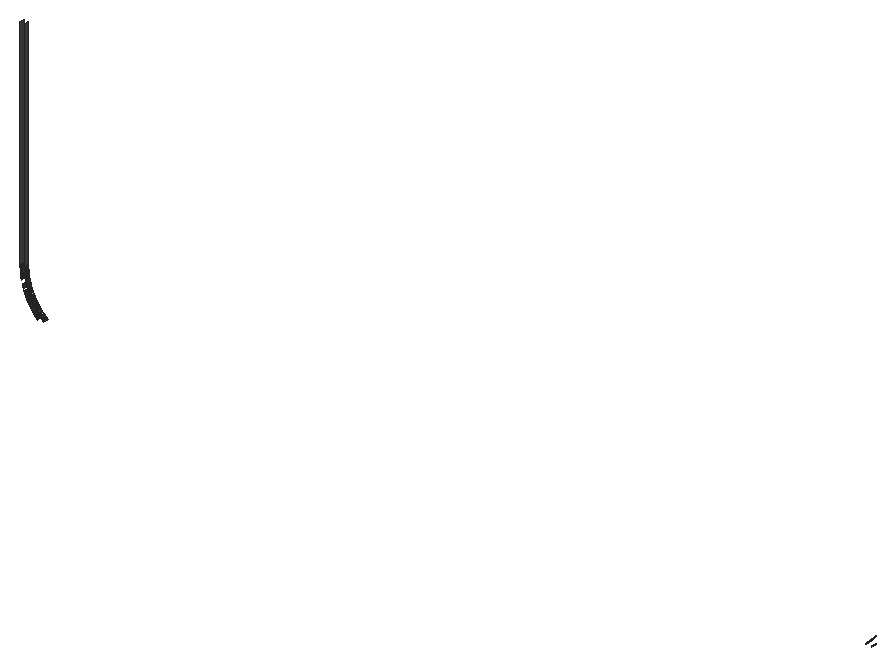
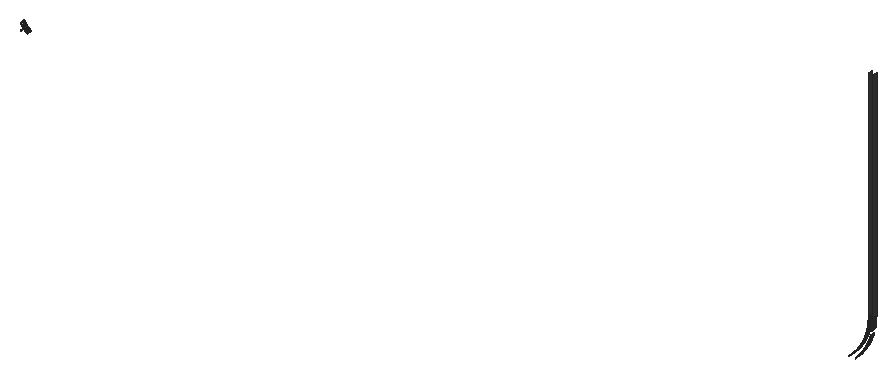
# SketchUp Ruby script. Lengths in inches.
U = 1.inch
M = Sketchup.active_model
def pt(a) = Geom::Point3d.new(a.map { |v| v * U })
def face(e, loops, mat)
  f = e.add_face(loops[0].map { |a| pt(a) })
  loops[1..].each { |l| e.add_face(l.map { |a| pt(a) }).erase! }
  f.material = f.back_material = mat if mat
  f
end
# faces: each face lists its corners as indices into pts; further lists are holes
def faces(e, pts, list, mat = nil) = list.each { |f| face(e, (f[0].is_a?(Array) ? f : [f]).map { |l| l.map { |i| pts[i] } }, mat) }
# xy, xz, yz: faces in a plane at the given z, y or x. An outline is a flat list of corners, or four numbers for a rectangle; further outlines are holes
def ring(l) = l.size == 4 ? [[l[0], l[1]], [l[2], l[1]], [l[2], l[3]], [l[0], l[3]]] : l.each_slice(2).to_a
def flat(e, list, mat, &to3) = list.each { |f| face(e, (f[0].is_a?(Array) ? f : [f]).map { |l| ring(l).map { |u, v| to3.(u, v) } }, mat) }
def xy(e, z, list, mat = nil) = flat(e, list, mat) { |x, y| [x, y, z] }
def xz(e, y, list, mat = nil) = flat(e, list, mat) { |x, z| [x, y, z] }
def yz(e, x, list, mat = nil) = flat(e, list, mat) { |y, z| [x, y, z] }
def lines(e, pts, list) = list.each { |a, b| e.add_line(pt(pts[a]), pt(pts[b])) }
# prism: a flat outline (further loops are holes) pulled along v
def prism(e, loops, v, mat = nil)
  f = face(e, loops, mat); d = Geom::Vector3d.new(v.map { |x| x * U })
  f.pushpull(f.normal.samedirection?(d) ? d.length : -d.length)
end
def box(e, o, s, mat = nil) = prism(e, [[o, [o[0] + s[0], o[1], o[2]], [o[0] + s[0], o[1] + s[1], o[2]], [o[0], o[1] + s[1], o[2]]]], [0, 0, s[2]], mat)
def at(x, y, z, deg = 0) = Geom::Transformation.translation(pt([x, y, z])) * Geom::Transformation.rotation(ORIGIN, Z_AXIS, deg.degrees)
def axes(o, x, y, z) = Geom::Transformation.new([*x, 0, *y, 0, *z, 0, *pt(o).to_a, 1])
def part(name) = M.definitions.add(name)
# library, detail: a bought-in or finely detailed component or shape, given as its bounding box
def library(name, o, s) = part(name).tap { |d| box(d.entities, o, s) }
def detail(e, o, s) = box(e.add_group.entities, o, s)
def put(e, d, t, mat = nil) = e.add_instance(d, t).tap { |i| i.material = mat if mat }
def group(e, t, mat = nil) = e.add_group.tap { |g| g.transformation = t; g.material = mat if mat }.entities
root = M.entities
M.materials.add("1432 AP 8245 TAR ROAD").color = [71, 72, 75]
M.materials.add("Outer Light").color = [251, 217, 152]
yz(root,258.5,[[95.37,191.47,96.87,191.63],[95.37,191.63,96.87,191.79],[95.37,191.79,96.87,266.79]],"1432 AP 8245 TAR ROAD")
yz(root,258.51,[[95.37,191.15,96.87,191.31]],"1432 AP 8245 TAR ROAD")
yz(root,258.52,[[95.37,190.83,96.87,190.99]],"1432 AP 8245 TAR ROAD")
yz(root,260,[[95.37,191.49,96.87,191.64],[95.37,191.64,96.87,191.79],[95.37,191.79,96.87,266.79]],"1432 AP 8245 TAR ROAD")
yz(root,260.01,[[95.37,191.05,96.87,191.2],[95.37,191.2,96.87,191.34]],"1432 AP 8245 TAR ROAD")
p = [[264.39,95.37,177.41],[264.5,95.37,177.3],[264.5,96.87,177.3],[264.39,96.87,177.41],[264.39,96.87,177.41],[264.5,96.87,177.3],
  [264.5,95.37,177.3],[264.39,95.37,177.41],[266.66,95.37,177.34],[266.55,95.37,177.44],[266.55,96.87,177.44],[266.66,96.87,177.34],
  [266.66,96.87,177.34],[266.55,96.87,177.44],[266.55,95.37,177.44],[266.66,95.37,177.34],[549.45,95.37,177.44],[549.34,95.37,177.34],
  [549.34,96.87,177.34],[549.45,96.87,177.44],[549.45,96.87,177.44],[549.34,96.87,177.34],[549.34,95.37,177.34],[549.45,95.37,177.44],
  [551.5,95.37,177.3],[551.61,95.37,177.41],[551.61,96.87,177.41],[551.5,96.87,177.3],[551.5,96.87,177.3],[551.61,96.87,177.41],
  [551.61,95.37,177.41],[551.5,95.37,177.3],[264.28,95.37,177.53],[264.28,96.87,177.53],[264.28,96.87,177.53],[264.28,95.37,177.53],
  [266.44,95.37,177.54],[266.44,96.87,177.54],[266.44,96.87,177.54],[266.44,95.37,177.54],[549.56,95.37,177.54],[549.56,96.87,177.54],
  [549.56,96.87,177.54],[549.56,95.37,177.54],[551.72,95.37,177.53],[551.72,96.87,177.53],[551.72,96.87,177.53],[551.72,95.37,177.53],
  [264.17,95.37,177.64],[264.17,96.87,177.64],[264.17,96.87,177.64],[264.17,95.37,177.64],[266.32,95.37,177.64],[266.32,96.87,177.64],
  [266.32,96.87,177.64],[266.32,95.37,177.64],[549.68,95.37,177.64],[549.68,96.87,177.64],[549.68,96.87,177.64],[549.68,95.37,177.64],
  [551.83,95.37,177.64],[551.83,96.87,177.64],[551.83,96.87,177.64],[551.83,95.37,177.64],[264.06,95.37,177.76],[264.06,96.87,177.76],
  [264.06,96.87,177.76],[264.06,95.37,177.76],[266.21,95.37,177.74],[266.21,96.87,177.74],[266.21,96.87,177.74],[266.21,95.37,177.74],
  [549.79,95.37,177.74],[549.79,96.87,177.74],[549.79,96.87,177.74],[549.79,95.37,177.74],[266.1,95.37,177.84],[266.1,96.87,177.84],
  [266.1,96.87,177.84],[266.1,95.37,177.84],[549.9,95.37,177.84],[549.9,96.87,177.84],[549.9,96.87,177.84],[549.9,95.37,177.84],
  [263.95,95.37,177.875],[263.95,96.87,177.875],[263.95,96.87,177.875],[263.95,95.37,177.875],[265.99,95.37,177.94],[265.99,96.87,177.94],
  [265.99,96.87,177.94],[265.99,95.37,177.94],[550.01,95.37,177.94],[550.01,96.87,177.94],[550.01,96.87,177.94],[550.01,95.37,177.94],
  [263.84,95.37,178],[263.84,96.87,178],[263.84,96.87,178],[263.84,95.37,178],[265.89,95.37,178.04],[265.89,96.87,178.04],
  [265.89,96.87,178.04],[265.89,95.37,178.04],[550.11,95.37,178.04],[550.11,96.87,178.04],[550.11,96.87,178.04],[550.11,95.37,178.04],
  [263.73,95.37,178.11],[263.73,96.87,178.11],[263.73,96.87,178.11],[263.73,95.37,178.11],[265.78,95.37,178.15],[265.78,96.87,178.15],
  [265.78,96.87,178.15],[265.78,95.37,178.15],[550.22,95.37,178.15],[550.22,96.87,178.15],[550.22,96.87,178.15],[550.22,95.37,178.15],
  [263.62,95.37,178.24],[263.62,96.87,178.24],[263.62,96.87,178.24],[263.62,95.37,178.24],[265.67,95.37,178.25],[265.67,96.87,178.25],
  [265.67,96.87,178.25],[265.67,95.37,178.25],[550.33,95.37,178.25],[550.33,96.87,178.25],[550.33,96.87,178.25],[550.33,95.37,178.25],
  [263.52,95.37,178.36],[263.52,96.87,178.36],[263.52,96.87,178.36],[263.52,95.37,178.36],[265.56,95.37,178.36],[265.56,96.87,178.36],
  [265.56,96.87,178.36],[265.56,95.37,178.36],[550.44,95.37,178.36],[550.44,96.87,178.36],[550.44,96.87,178.36],[550.44,95.37,178.36],
  [263.41,95.37,178.48],[263.41,96.87,178.48],[263.41,96.87,178.48],[263.41,95.37,178.48],[265.46,95.37,178.46],[265.46,96.87,178.46],
  [265.46,96.87,178.46],[265.46,95.37,178.46],[550.54,95.37,178.46],[550.54,96.87,178.46],[550.54,96.87,178.46],[550.54,95.37,178.46],
  [263.31,95.37,178.6],[263.31,96.87,178.6],[263.31,96.87,178.6],[263.31,95.37,178.6],[265.36,95.37,178.57],[265.36,96.87,178.57],
  [265.36,96.87,178.57],[265.36,95.37,178.57],[550.64,95.37,178.57],[550.64,96.87,178.57],[550.64,96.87,178.57],[550.64,95.37,178.57],
  [263.2,95.37,178.72],[263.2,96.87,178.72],[263.2,96.87,178.72],[263.2,95.37,178.72],[265.25,95.37,178.68],[265.25,96.87,178.68],
  [265.25,96.87,178.68],[265.25,95.37,178.68],[550.75,95.37,178.68],[550.75,96.87,178.68],[550.75,96.87,178.68],[550.75,95.37,178.68],
  [263.1,95.37,178.85],[263.1,96.87,178.85],[263.1,96.87,178.85],[263.1,95.37,178.85],[265.15,95.37,178.79],[265.15,96.87,178.79],
  [265.15,96.87,178.79],[265.15,95.37,178.79],[550.85,95.37,178.79],[550.85,96.87,178.79],[550.85,96.87,178.79],[550.85,95.37,178.79],
  [263,95.37,178.97],[263,96.87,178.97],[263,96.87,178.97],[263,95.37,178.97],[265.05,95.37,178.89],[265.05,96.87,178.89],
  [265.05,96.87,178.89],[265.05,95.37,178.89],[550.95,95.37,178.89],[550.95,96.87,178.89],[550.95,96.87,178.89],[550.95,95.37,178.89],
  [264.95,95.37,179],[264.95,96.87,179],[264.95,96.87,179],[264.95,95.37,179],[551.05,95.37,179],[551.05,96.87,179],
  [551.05,96.87,179],[551.05,95.37,179],[262.9,95.37,179.1],[262.9,96.87,179.1],[262.9,96.87,179.1],[262.9,95.37,179.1],
  [264.85,95.37,179.12],[264.85,96.87,179.12],[264.85,96.87,179.12],[264.85,95.37,179.12],[551.15,95.37,179.12],[551.15,96.87,179.12],
  [551.15,96.87,179.12],[551.15,95.37,179.12],[262.8,95.37,179.23],[262.8,96.87,179.23],[262.8,96.87,179.23],[262.8,95.37,179.23],
  [264.75,95.37,179.23],[264.75,96.87,179.23],[264.75,96.87,179.23],[264.75,95.37,179.23],[551.25,95.37,179.23],[551.25,96.87,179.23],
  [551.25,96.87,179.23],[551.25,95.37,179.23],[262.7,95.37,179.36],[262.7,96.87,179.36],[262.7,96.87,179.36],[262.7,95.37,179.36],
  [264.65,95.37,179.34],[264.65,96.87,179.34],[264.65,96.87,179.34],[264.65,95.37,179.34],[551.35,95.37,179.34],[551.35,96.87,179.34],
  [551.35,96.87,179.34],[551.35,95.37,179.34],[264.55,95.37,179.45],[264.55,96.87,179.45],[264.55,96.87,179.45],[264.55,95.37,179.45],
  [551.45,95.37,179.45],[551.45,96.87,179.45],[551.45,96.87,179.45],[551.45,95.37,179.45],[262.61,95.37,179.48],[262.61,96.87,179.48],
  [262.61,96.87,179.48],[262.61,95.37,179.48],[262.51,95.37,179.61],[262.51,96.87,179.61],[262.51,96.87,179.61],[262.51,95.37,179.61],
  [264.46,95.37,179.57],[264.46,96.87,179.57],[264.46,96.87,179.57],[264.46,95.37,179.57],[551.54,95.37,179.57],[551.54,96.87,179.57],
  [551.54,96.87,179.57],[551.54,95.37,179.57],[262.42,95.37,179.74],[262.42,96.87,179.74],[262.42,96.87,179.74],[262.42,95.37,179.74],
  [264.36,95.37,179.68],[264.36,96.87,179.68],[264.36,96.87,179.68],[264.36,95.37,179.68],[551.64,95.37,179.68],[551.64,96.87,179.68],
  [551.64,96.87,179.68],[551.64,95.37,179.68],[262.32,95.37,179.875],[262.32,96.87,179.875],[262.32,96.87,179.875],[262.32,95.37,179.875],
  [264.27,95.37,179.8],[264.27,96.87,179.8],[264.27,96.87,179.8],[264.27,95.37,179.8],[551.73,95.37,179.8],[551.73,96.87,179.8],
  [551.73,96.87,179.8],[551.73,95.37,179.8],[264.17,95.37,179.91],[264.17,96.87,179.91],[264.17,96.87,179.91],[264.17,95.37,179.91],
  [551.83,95.37,179.91],[551.83,96.87,179.91],[551.83,96.87,179.91],[551.83,95.37,179.91],[262.23,95.37,180],[262.23,96.87,180],
  [262.23,96.87,180],[262.23,95.37,180],[264.08,95.37,180.03],[264.08,96.87,180.03],[264.08,96.87,180.03],[264.08,95.37,180.03],
  [262.14,95.37,180.14],[262.14,96.87,180.14],[262.14,96.87,180.14],[262.14,95.37,180.14],[263.99,95.37,180.15],[263.99,96.87,180.15],
  [263.99,96.87,180.15],[263.99,95.37,180.15],[262.04,95.37,180.27],[262.04,96.87,180.27],[262.04,96.87,180.27],[262.04,95.37,180.27],
  [263.9,95.37,180.27],[263.9,96.87,180.27],[263.9,96.87,180.27],[263.9,95.37,180.27],[261.95,95.37,180.4],[261.95,96.87,180.4],
  [261.95,96.87,180.4],[261.95,95.37,180.4],[263.81,95.37,180.38],[263.81,96.87,180.38],[263.81,96.87,180.38],[263.81,95.37,180.38],
  [261.87,95.37,180.54],[261.87,96.87,180.54],[261.87,96.87,180.54],[261.87,95.37,180.54],[263.72,95.37,180.5],[263.72,96.87,180.5],
  [263.72,96.87,180.5],[263.72,95.37,180.5],[261.78,95.37,180.67],[261.78,96.87,180.67],[261.78,96.87,180.67],[261.78,95.37,180.67],
  [263.63,95.37,180.625],[263.63,96.87,180.625],[263.63,96.87,180.625],[263.63,95.37,180.625],[263.54,95.37,180.75],[263.54,96.87,180.75],
  [263.54,96.87,180.75],[263.54,95.37,180.75],[261.69,95.37,180.81],[261.69,96.87,180.81],[261.69,96.87,180.81],[261.69,95.37,180.81],
  [263.46,95.37,180.87],[263.46,96.87,180.87],[263.46,96.87,180.87],[263.46,95.37,180.87],[261.61,95.37,180.94],[261.61,96.87,180.94],
  [261.61,96.87,180.94],[261.61,95.37,180.94],[261.52,95.37,181.08],[261.52,96.87,181.08],[261.52,96.87,181.08],[261.52,95.37,181.08],
  [263.37,95.37,180.99],[263.37,96.87,180.99],[263.37,96.87,180.99],[263.37,95.37,180.99],[263.29,95.37,181.11],[263.29,96.87,181.11],
  [263.29,96.87,181.11],[263.29,95.37,181.11],[261.4375,95.37,181.22],[261.4375,96.87,181.22],[261.4375,96.87,181.22],[261.4375,95.37,181.22],
  [263.2,95.37,181.24],[263.2,96.87,181.24],[263.2,96.87,181.24],[263.2,95.37,181.24],[261.35,95.37,181.36],[261.35,96.87,181.36],
  [261.35,96.87,181.36],[261.35,95.37,181.36],[263.12,95.37,181.36],[263.12,96.87,181.36],[263.12,96.87,181.36],[263.12,95.37,181.36],
  [261.27,95.37,181.5],[261.27,96.87,181.5],[261.27,96.87,181.5],[261.27,95.37,181.5],[263.04,95.37,181.49],[263.04,96.87,181.49],
  [263.04,96.87,181.49],[263.04,95.37,181.49],[261.19,95.37,181.64],[261.19,96.87,181.64],[261.19,96.87,181.64],[261.19,95.37,181.64],
  [262.96,95.37,181.61],[262.96,96.87,181.61],[262.96,96.87,181.61],[262.96,95.37,181.61],[261.11,95.37,181.78],[261.11,96.87,181.78],
  [261.11,96.87,181.78],[261.11,95.37,181.78],[262.88,95.37,181.74],[262.88,96.87,181.74],[262.88,96.87,181.74],[262.88,95.37,181.74],
  [262.8,95.37,181.86],[262.8,96.87,181.86],[262.8,96.87,181.86],[262.8,95.37,181.86],[261.04,95.37,181.92],[261.04,96.87,181.92],
  [261.04,96.87,181.92],[261.04,95.37,181.92],[260.96,95.37,182.06],[260.96,96.87,182.06],[260.96,96.87,182.06],[260.96,95.37,182.06],
  [262.72,95.37,181.99],[262.72,96.87,181.99],[262.72,96.87,181.99],[262.72,95.37,181.99],[262.65,95.37,182.12],[262.65,96.87,182.12],
  [262.65,96.87,182.12],[262.65,95.37,182.12],[260.88,95.37,182.2],[260.88,96.87,182.2],[260.88,96.87,182.2],[260.88,95.37,182.2],
  [262.57,95.37,182.25],[262.57,96.87,182.25],[262.57,96.87,182.25],[262.57,95.37,182.25],[260.81,95.37,182.34],[260.81,96.87,182.34],
  [260.81,96.87,182.34],[260.81,95.37,182.34],[262.5,95.37,182.38],[262.5,96.87,182.38],[262.5,96.87,182.38],[262.5,95.37,182.38],
  [260.73,95.37,182.49],[260.73,96.87,182.49],[260.73,96.87,182.49],[260.73,95.37,182.49],[262.42,95.37,182.51],[262.42,96.87,182.51],
  [262.42,96.87,182.51],[262.42,95.37,182.51],[260.66,95.37,182.63],[260.66,96.87,182.63],[260.66,96.87,182.63],[260.66,95.37,182.63],
  [262.35,95.37,182.64],[262.35,96.87,182.64],[262.35,96.87,182.64],[262.35,95.37,182.64],[260.59,95.37,182.77],[260.59,96.87,182.77],
  [260.59,96.87,182.77],[260.59,95.37,182.77],[262.28,95.37,182.77],[262.28,96.87,182.77],[262.28,96.87,182.77],[262.28,95.37,182.77],
  [260.52,95.37,182.92],[260.52,96.87,182.92],[260.52,96.87,182.92],[260.52,95.37,182.92],[262.21,95.37,182.9],[262.21,96.87,182.9],
  [262.21,96.87,182.9],[262.21,95.37,182.9],[260.45,95.37,183.0625],[260.45,96.87,183.0625],[260.45,96.87,183.0625],[260.45,95.37,183.0625],
  [262.14,95.37,183.03],[262.14,96.87,183.03],[262.14,96.87,183.03],[262.14,95.37,183.03],[262.07,95.37,183.17],[262.07,96.87,183.17],
  [262.07,96.87,183.17],[262.07,95.37,183.17],[260.38,95.37,183.21],[260.38,96.87,183.21],[260.38,96.87,183.21],[260.38,95.37,183.21],
  [260.32,95.37,183.36],[260.32,96.87,183.36],[260.32,96.87,183.36],[260.32,95.37,183.36],[262,95.37,183.3],[262,96.87,183.3],
  [262,96.87,183.3],[262,95.37,183.3],[261.9375,95.37,183.43],[261.9375,96.87,183.43],[261.9375,96.87,183.43],[261.9375,95.37,183.43],
  [260.25,95.37,183.5],[260.25,96.87,183.5],[260.25,96.87,183.5],[260.25,95.37,183.5],[261.87,95.37,183.57],[261.87,96.87,183.57],
  [261.87,96.87,183.57],[261.87,95.37,183.57],[260.1875,95.37,183.65],[260.1875,96.87,183.65],[260.1875,96.87,183.65],[260.1875,95.37,183.65],
  [261.81,95.37,183.7],[261.81,96.87,183.7],[261.81,96.87,183.7],[261.81,95.37,183.7],[260.12,95.37,183.8],[260.12,96.87,183.8],
  [260.12,96.87,183.8],[260.12,95.37,183.8],[261.75,95.37,183.84],[261.75,96.87,183.84],[261.75,96.87,183.84],[261.75,95.37,183.84],
  [260.06,95.37,183.95],[260.06,96.87,183.95],[260.06,96.87,183.95],[260.06,95.37,183.95],[261.68,95.37,183.97],[261.68,96.87,183.97],
  [261.68,96.87,183.97],[261.68,95.37,183.97],[260,95.37,184.1],[260,96.87,184.1],[260,96.87,184.1],[260,95.37,184.1],
  [261.62,95.37,184.11],[261.62,96.87,184.11],[261.62,96.87,184.11],[261.62,95.37,184.11],[259.94,95.37,184.25],[259.94,96.87,184.25],
  [259.94,96.87,184.25],[259.94,95.37,184.25],[261.5625,95.37,184.25],[261.5625,96.87,184.25],[261.5625,96.87,184.25],[261.5625,95.37,184.25],
  [259.88,95.37,184.4],[259.88,96.87,184.4],[259.88,96.87,184.4],[259.88,95.37,184.4],[261.5,95.37,184.38],[261.5,96.87,184.38],
  [261.5,96.87,184.38],[261.5,95.37,184.38],[259.82,95.37,184.55],[259.82,96.87,184.55],[259.82,96.87,184.55],[259.82,95.37,184.55],
  [261.45,95.37,184.52],[261.45,96.87,184.52],[261.45,96.87,184.52],[261.45,95.37,184.52],[261.39,95.37,184.66],[261.39,96.87,184.66],
  [261.39,96.87,184.66],[261.39,95.37,184.66],[261.33,95.37,184.8],[261.33,96.87,184.8],[261.28,95.37,184.9375],[261.28,96.87,184.9375],
  [261.23,95.37,185.08],[261.23,96.87,185.08],[259.61,95.37,185.15],[259.66,95.37,185],[259.66,96.87,185],[259.61,96.87,185.15],
  [261.17,95.37,185.22],[261.17,96.87,185.22],[259.55,95.37,185.3],[259.55,96.87,185.3],[261.125,95.37,185.36],[261.125,96.87,185.36],
  [259.5,95.37,185.46],[259.5,96.87,185.46],[261.07,95.37,185.5],[261.07,96.87,185.5],[259.45,95.37,185.61],[259.45,96.87,185.61],
  [261.02,95.37,185.64],[261.02,96.87,185.64],[259.41,95.37,185.76],[259.41,96.87,185.76],[260.98,95.37,185.78],[260.98,96.87,185.78],
  [259.36,95.37,185.92],[259.36,96.87,185.92],[260.93,95.37,185.92],[260.93,96.87,185.92],[259.3125,95.37,186.07],[259.3125,96.87,186.07],
  [260.88,95.37,186.0625],[260.88,96.87,186.0625],[259.27,95.37,186.23],[259.27,96.87,186.23],[260.84,95.37,186.21],[260.84,96.87,186.21],
  [259.23,95.37,186.38],[259.23,96.87,186.38],[260.8,95.37,186.35],[260.8,96.87,186.35],[260.75,95.37,186.49],[260.75,96.87,186.49],
  [260.71,95.37,186.63],[260.71,96.87,186.63],[260.67,95.37,186.78],[260.67,96.87,186.78],[260.63,95.37,186.92],[260.63,96.87,186.92],
  [260.6,95.37,187.07],[260.6,96.87,187.07],[260.56,95.37,187.21],[260.56,96.87,187.21],[260.52,95.37,187.36],[260.52,96.87,187.36],
  [260.49,95.37,187.5],[260.49,96.87,187.5],[260.46,95.37,187.65],[260.46,96.87,187.65],[258.89,95.37,187.79],[258.93,95.37,187.63],
  [258.93,96.87,187.63],[258.89,96.87,187.79],[260.43,95.37,187.79],[260.43,96.87,187.79],[258.86,95.37,187.95],[258.86,96.87,187.95],
  [260.39,95.37,187.9375],[260.39,96.87,187.9375],[260.37,95.37,188.09],[260.37,96.87,188.09],[258.83,95.37,188.11],[258.83,96.87,188.11],
  [258.81,95.37,188.27],[258.81,96.87,188.27],[260.34,95.37,188.23],[260.34,96.87,188.23],[260.31,95.37,188.38],[260.31,96.87,188.38],
  [258.78,95.37,188.43],[258.78,96.87,188.43],[258.75,95.37,188.59],[258.75,96.87,188.59],[260.28,95.37,188.53],[260.28,96.87,188.53],
  [260.26,95.37,188.67],[260.26,96.87,188.67],[258.73,95.37,188.74],[258.73,96.87,188.74],[258.7,95.37,188.9],[258.7,96.87,188.9],
  [260.23,95.37,188.82],[260.23,96.87,188.82],[260.21,95.37,188.97],[260.21,96.87,188.97],[258.68,95.37,189.0625],[258.68,96.87,189.0625],
  [260.19,95.37,189.11],[260.19,96.87,189.11],[258.66,95.37,189.22],[258.66,96.87,189.22],[260.17,95.37,189.26],[260.17,96.87,189.26],
  [258.64,95.37,189.38],[258.64,96.87,189.38],[260.15,95.37,189.41],[260.15,96.87,189.41],[258.625,95.37,189.54],[258.625,96.87,189.54],
  [260.13,95.37,189.56],[260.13,96.87,189.56],[258.61,95.37,189.7],[258.61,96.87,189.7],[260.11,95.37,189.71],[260.11,96.87,189.71],
  [258.59,95.37,189.86],[258.59,96.87,189.86],[260.1,95.37,189.86],[260.1,96.87,189.86],[258.58,95.37,190.02],[258.58,96.87,190.02],
  [260.08,95.37,190],[260.08,96.87,190],[258.5625,95.37,190.18],[258.5625,96.87,190.18],[260.07,95.37,190.15],[260.07,96.87,190.15],
  [258.55,95.37,190.34],[258.55,96.87,190.34],[260.06,95.37,190.3],[260.06,96.87,190.3],[258.54,95.37,190.5],[258.54,96.87,190.5],
  [260.05,95.37,190.45],[260.05,96.87,190.45],[258.53,95.37,190.67],[258.53,96.87,190.67],[260.04,95.37,190.6],[260.04,96.87,190.6],
  [260.03,95.37,190.75],[260.03,96.87,190.75],[258.52,95.37,190.83],[258.52,96.87,190.83],[260.02,95.37,190.9],[260.02,96.87,190.9],
  [260.01,95.37,191.05],[260.01,96.87,191.05],[258.51,95.37,191.15],[258.52,95.37,190.99],[258.52,96.87,190.99],[258.51,96.87,191.15],
  [258.5,95.37,191.47],[258.51,95.37,191.31],[258.51,96.87,191.31],[258.5,96.87,191.47],[260.01,95.37,191.34],[260,95.37,191.49],
  [260,96.87,191.49],[260.01,96.87,191.34]]
faces(root,p,[[0,1,2,3],[8,9,10,11],[16,17,18,19],[24,25,26,27],[32,0,3,33],[9,36,37,10],[40,16,19,41],[25,44,45,26],
  [48,32,33,49],[36,52,53,37],[56,40,41,57],[44,60,61,45],[64,48,49,65],[52,68,69,53],[72,56,57,73],[68,76,77,69],
  [80,72,73,81],[84,64,65,85],[76,88,89,77],[92,80,81,93],[96,84,85,97],[88,100,101,89],[104,92,93,105],[108,96,97,109],
  [100,112,113,101],[116,104,105,117],[120,108,109,121],[112,124,125,113],[128,116,117,129],[132,120,121,133],[124,136,137,125],[140,128,129,141],
  [144,132,133,145],[136,148,149,137],[152,140,141,153],[156,144,145,157],[148,160,161,149],[164,152,153,165],[168,156,157,169],[160,172,173,161],
  [176,164,165,177],[180,168,169,181],[172,184,185,173],[188,176,177,189],[192,180,181,193],[184,196,197,185],[200,188,189,201],[196,204,205,197],
  [208,200,201,209],[212,192,193,213],[204,216,217,205],[220,208,209,221],[224,212,213,225],[216,228,229,217],[232,220,221,233],[236,224,225,237],
  [228,240,241,229],[244,232,233,245],[240,248,249,241],[252,244,245,253],[256,236,237,257],[260,256,257,261],[248,264,265,249],[268,252,253,269],
  [272,260,261,273],[264,276,277,265],[280,268,269,281],[284,272,273,285],[276,288,289,277],[292,280,281,293],[288,296,297,289],[300,292,293,301],
  [304,284,285,305],[296,308,309,297],[312,304,305,313],[308,316,317,309],[320,312,313,321],[316,324,325,317],[328,320,321,329],[324,332,333,325],
  [336,328,329,337],[332,340,341,333],[344,336,337,345],[340,348,349,341],[348,352,353,349],[356,344,345,357],[352,360,361,353],[364,356,357,365],
  [368,364,365,369],[360,372,373,361],[372,376,377,373],[380,368,369,381],[376,384,385,377],[388,380,381,389],[384,392,393,385],[396,388,389,397],
  [392,400,401,393],[404,396,397,405],[400,408,409,401],[412,404,405,413],[408,416,417,409],[416,420,421,417],[424,412,413,425],[428,424,425,429],
  [420,432,433,421],[432,436,437,433],[440,428,429,441],[436,444,445,437],[448,440,441,449],[444,452,453,445],[456,448,449,457],[452,460,461,453],
  [464,456,457,465],[460,468,469,461],[472,464,465,473],[468,476,477,469],[480,472,473,481],[476,484,485,477],[488,480,481,489],[484,492,493,485],
  [492,496,497,493],[500,488,489,501],[504,500,501,505],[496,508,509,497],[508,512,513,509],[516,504,505,517],[512,520,521,513],[524,516,517,525],
  [520,528,529,521],[532,524,525,533],[528,536,537,529],[540,532,533,541],[536,544,545,537],[548,540,541,549],[544,552,553,545],[556,548,549,557],
  [552,560,561,553],[564,556,557,565],[560,568,569,561],[572,564,565,573],[568,576,577,569],[576,580,581,577],[580,584,585,581],[584,586,587,585],
  [586,588,589,587],[590,591,592,593],[588,594,595,589],[596,590,593,597],[594,598,599,595],[600,596,597,601],[598,602,603,599],[604,600,601,605],
  [602,606,607,603],[608,604,605,609],[606,610,611,607],[612,608,609,613],[610,614,615,611],[616,612,613,617],[614,618,619,615],[620,616,617,621],
  [618,622,623,619],[624,620,621,625],[622,626,627,623],[626,628,629,627],[628,630,631,629],[630,632,633,631],[632,634,635,633],[634,636,637,635],
  [636,638,639,637],[638,640,641,639],[640,642,643,641],[642,644,645,643],[646,647,648,649],[644,650,651,645],[652,646,649,653],[650,654,655,651],
  [654,656,657,655],[658,652,653,659],[660,658,659,661],[656,662,663,657],[662,664,665,663],[666,660,661,667],[668,666,667,669],[664,670,671,665],
  [670,672,673,671],[674,668,669,675],[676,674,675,677],[672,678,679,673],[678,680,681,679],[682,676,677,683],[680,684,685,681],[686,682,683,687],
  [684,688,689,685],[690,686,687,691],[688,692,693,689],[694,690,691,695],[692,696,697,693],[698,694,695,699],[696,700,701,697],[702,698,699,703],
  [700,704,705,701],[706,702,703,707],[704,708,709,705],[710,706,707,711],[708,712,713,709],[714,710,711,715],[712,716,717,713],[718,714,715,719],
  [716,720,721,717],[722,718,719,723],[720,724,725,721],[724,726,727,725],[728,722,723,729],[726,730,731,727],[730,732,733,731],[734,735,736,737],
  [738,739,740,741],[742,743,744,745]],"1432 AP 8245 TAR ROAD")
faces(root,p,[[4,5,6,7],[12,13,14,15],[20,21,22,23],[28,29,30,31],[34,4,7,35],[13,38,39,14],[42,20,23,43],[29,46,47,30],
  [50,34,35,51],[38,54,55,39],[58,42,43,59],[46,62,63,47],[66,50,51,67],[54,70,71,55],[74,58,59,75],[70,78,79,71],
  [82,74,75,83],[86,66,67,87],[78,90,91,79],[94,82,83,95],[98,86,87,99],[90,102,103,91],[106,94,95,107],[110,98,99,111],
  [102,114,115,103],[118,106,107,119],[122,110,111,123],[114,126,127,115],[130,118,119,131],[134,122,123,135],[126,138,139,127],[142,130,131,143],
  [146,134,135,147],[138,150,151,139],[154,142,143,155],[158,146,147,159],[150,162,163,151],[166,154,155,167],[170,158,159,171],[162,174,175,163],
  [178,166,167,179],[182,170,171,183],[174,186,187,175],[190,178,179,191],[194,182,183,195],[186,198,199,187],[202,190,191,203],[198,206,207,199],
  [210,202,203,211],[214,194,195,215],[206,218,219,207],[222,210,211,223],[226,214,215,227],[218,230,231,219],[234,222,223,235],[238,226,227,239],
  [230,242,243,231],[246,234,235,247],[242,250,251,243],[254,246,247,255],[258,238,239,259],[262,258,259,263],[250,266,267,251],[270,254,255,271],
  [274,262,263,275],[266,278,279,267],[282,270,271,283],[286,274,275,287],[278,290,291,279],[294,282,283,295],[290,298,299,291],[302,294,295,303],
  [306,286,287,307],[298,310,311,299],[314,306,307,315],[310,318,319,311],[322,314,315,323],[318,326,327,319],[330,322,323,331],[326,334,335,327],
  [338,330,331,339],[334,342,343,335],[346,338,339,347],[342,350,351,343],[350,354,355,351],[358,346,347,359],[354,362,363,355],[366,358,359,367],
  [370,366,367,371],[362,374,375,363],[374,378,379,375],[382,370,371,383],[378,386,387,379],[390,382,383,391],[386,394,395,387],[398,390,391,399],
  [394,402,403,395],[406,398,399,407],[402,410,411,403],[414,406,407,415],[410,418,419,411],[418,422,423,419],[426,414,415,427],[430,426,427,431],
  [422,434,435,423],[434,438,439,435],[442,430,431,443],[438,446,447,439],[450,442,443,451],[446,454,455,447],[458,450,451,459],[454,462,463,455],
  [466,458,459,467],[462,470,471,463],[474,466,467,475],[470,478,479,471],[482,474,475,483],[478,486,487,479],[490,482,483,491],[486,494,495,487],
  [494,498,499,495],[502,490,491,503],[506,502,503,507],[498,510,511,499],[510,514,515,511],[518,506,507,519],[514,522,523,515],[526,518,519,527],
  [522,530,531,523],[534,526,527,535],[530,538,539,531],[542,534,535,543],[538,546,547,539],[550,542,543,551],[546,554,555,547],[558,550,551,559],
  [554,562,563,555],[566,558,559,567],[562,570,571,563],[574,566,567,575],[570,578,579,571],[578,582,583,579]],"Outer Light")
